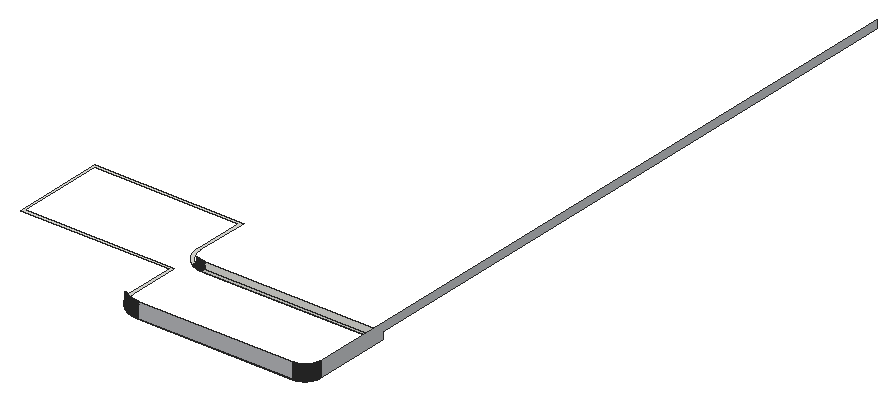
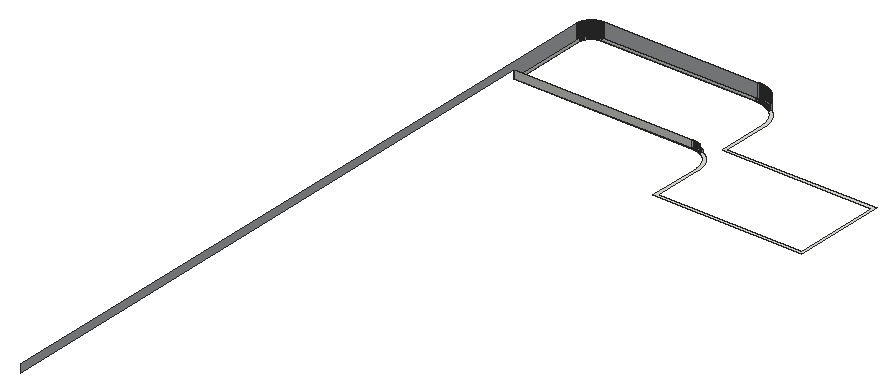
# SketchUp Ruby script. Lengths in inches.
U = 1.inch
M = Sketchup.active_model
def pt(a) = Geom::Point3d.new(a.map { |v| v * U })
def face(e, loops, mat)
  f = e.add_face(loops[0].map { |a| pt(a) })
  loops[1..].each { |l| e.add_face(l.map { |a| pt(a) }).erase! }
  f.material = f.back_material = mat if mat
  f
end
# faces: each face lists its corners as indices into pts; further lists are holes
def faces(e, pts, list, mat = nil) = list.each { |f| face(e, (f[0].is_a?(Array) ? f : [f]).map { |l| l.map { |i| pts[i] } }, mat) }
# xy, xz, yz: faces in a plane at the given z, y or x. An outline is a flat list of corners, or four numbers for a rectangle; further outlines are holes
def ring(l) = l.size == 4 ? [[l[0], l[1]], [l[2], l[1]], [l[2], l[3]], [l[0], l[3]]] : l.each_slice(2).to_a
def flat(e, list, mat, &to3) = list.each { |f| face(e, (f[0].is_a?(Array) ? f : [f]).map { |l| ring(l).map { |u, v| to3.(u, v) } }, mat) }
def xy(e, z, list, mat = nil) = flat(e, list, mat) { |x, y| [x, y, z] }
def xz(e, y, list, mat = nil) = flat(e, list, mat) { |x, z| [x, y, z] }
def yz(e, x, list, mat = nil) = flat(e, list, mat) { |y, z| [x, y, z] }
def lines(e, pts, list) = list.each { |a, b| e.add_line(pt(pts[a]), pt(pts[b])) }
# prism: a flat outline (further loops are holes) pulled along v
def prism(e, loops, v, mat = nil)
  f = face(e, loops, mat); d = Geom::Vector3d.new(v.map { |x| x * U })
  f.pushpull(f.normal.samedirection?(d) ? d.length : -d.length)
end
def box(e, o, s, mat = nil) = prism(e, [[o, [o[0] + s[0], o[1], o[2]], [o[0] + s[0], o[1] + s[1], o[2]], [o[0], o[1] + s[1], o[2]]]], [0, 0, s[2]], mat)
def at(x, y, z, deg = 0) = Geom::Transformation.translation(pt([x, y, z])) * Geom::Transformation.rotation(ORIGIN, Z_AXIS, deg.degrees)
def axes(o, x, y, z) = Geom::Transformation.new([*x, 0, *y, 0, *z, 0, *pt(o).to_a, 1])
def part(name) = M.definitions.add(name)
# library, detail: a bought-in or finely detailed component or shape, given as its bounding box
def library(name, o, s) = part(name).tap { |d| box(d.entities, o, s) }
def detail(e, o, s) = box(e.add_group.entities, o, s)
def put(e, d, t, mat = nil) = e.add_instance(d, t).tap { |i| i.material = mat if mat }
def group(e, t, mat = nil) = e.add_group.tap { |g| g.transformation = t; g.material = mat if mat }.entities
root = M.entities
M.materials.add("1427 AP 686 ARMOUR-N").color = [184, 186, 189]
xy(root,114,[[[157.6875,120,157.37,120.01,157.06,120.02,156.74,120.03,156.12,120.07,155.8,120.1,155.49,120.13,154.56,120.25,154.25,120.3,153.625,120.4,153.32,120.46,153.01,120.52,152.7,120.59,152.4,120.66,152.09,120.74,151.49,120.9,151.18,120.99,150.58,121.17,150.29,121.27,149.69,121.48,149.4,121.59,148.24,122.07,147.95,122.2,147.39,122.48,147.1,122.62,146.83,122.76,146.27,123.06,146,123.22,145.73,123.375,145.46,123.54,145.19,123.7,144.67,124.04,143.89,124.58,143.14,125.15,142.9,125.35,142.65,125.55,142.41,125.75,142.18,125.96,141.94,126.16,141.48,126.59,141.25,126.81,140.81,127.25,140.59,127.48,140.16,127.94,139.96,128.18,139.75,128.41,139.55,128.65,139.35,128.9,139.15,129.14,138.58,129.89,138.04,130.67,137.7,131.19,137.54,131.46,137.375,131.73,137.22,132,137.06,132.27,136.76,132.83,136.62,133.1,136.48,133.39,136.2,133.95,136.07,134.24,135.59,135.4,135.48,135.69,135.27,136.29,135.17,136.58,134.99,137.18,134.9,137.49,134.74,138.09,134.66,138.4,134.59,138.7,134.52,139.01,134.46,139.32,134.4,139.625,134.3,140.25,134.25,140.56,134.13,141.49,134.1,141.8,134.07,142.12,134.03,142.74,134.02,143.06,134.01,143.37,134,143.6875,134,180,18,180,18,252,134,252,134,209.78,134.01,209.57,134.01,209.35,134.03,208.91,134.05,208.7,134.0625,208.48,134.08,208.26,134.11,208.05,134.13,207.83,134.16,207.61,134.1875,207.4,134.22,207.18,134.26,206.97,134.29,206.76,134.34,206.54,134.42,206.12,134.47,205.9,134.52,205.69,134.58,205.48,134.63,205.27,134.69,205.0625,134.75,204.85,134.82,204.64,134.88,204.4375,134.95,204.23,135.02,204.03,135.09,203.82,135.17,203.62,135.25,203.41,135.41,203.01,135.5,202.8125,135.59,202.61,135.68,202.41,135.77,202.22,135.86,202.02,135.96,201.83,136.0625,201.63,136.16,201.44,136.27,201.25,136.48,200.875,136.6,200.6875,136.71,200.5,136.83,200.32,136.94,200.14,137.0625,199.95,137.1875,199.77,137.3125,199.6,137.4375,199.42,137.57,199.24,137.83,198.9,137.97,198.73,138.1,198.56,138.24,198.39,138.38,198.23,138.53,198.0625,138.67,197.9,138.97,197.58,139.12,197.43,139.27,197.27,139.43,197.12,139.58,196.97,139.9,196.67,140.0625,196.53,140.23,196.38,140.39,196.24,140.56,196.1,140.73,195.97,140.9,195.83,141.24,195.57,141.42,195.4375,141.6,195.3125,141.77,195.1875,141.95,195.0625,142.14,194.94,142.32,194.83,142.5,194.71,142.6875,194.6,142.875,194.48,143.25,194.27,143.44,194.16,143.63,194.0625,143.83,193.96,144.02,193.86,144.22,193.77,144.41,193.68,144.61,193.59,144.8125,193.5,145.01,193.41,145.41,193.25,145.62,193.17,145.82,193.09,146.03,193.02,146.23,192.95,146.4375,192.88,146.64,192.82,146.85,192.75,147.0625,192.69,147.27,192.63,147.48,192.58,147.69,192.52,147.9,192.47,148.12,192.42,148.54,192.34,148.76,192.29,148.97,192.26,149.18,192.22,149.4,192.1875,149.61,192.16,149.83,192.13,150.05,192.11,150.26,192.08,150.48,192.0625,150.7,192.05,150.91,192.03,151.35,192.01,151.57,192.01,151.78,192,290,192,290,131.76,289.99,131.53,289.98,131.29,289.96,131.06,289.94,130.82,289.92,130.59,289.89,130.36,289.85,130.12,289.8125,129.89,289.77,129.66,289.67,129.2,289.55,128.74,289.48,128.52,289.41,128.29,289.34,128.07,289.26,127.85,289.17,127.625,289.09,127.41,288.99,127.19,288.9,126.98,288.8,126.76,288.58,126.34,288.47,126.14,288.35,125.93,288.11,125.53,287.98,125.33,287.84,125.14,287.71,124.95,287.57,124.76,287.42,124.57,287.28,124.39,286.97,124.03,286.8125,123.85,286.65,123.68,286.49,123.51,286.32,123.35,286.15,123.1875,285.97,123.03,285.61,122.72,285.43,122.58,285.24,122.43,285.05,122.29,284.86,122.16,284.67,122.02,284.47,121.89,284.07,121.65,283.86,121.53,283.66,121.42,283.24,121.2,283.02,121.1,282.81,121.01,282.59,120.91,282.375,120.83,282.15,120.74,281.93,120.66,281.71,120.59,281.48,120.52,281.26,120.45,280.8,120.33,280.34,120.23,280.11,120.1875,279.88,120.15,279.64,120.11,279.41,120.08,279.18,120.06,278.94,120.04,278.71,120.02,278.47,120.01,278.24,120],[157.71,122,278.2,122,278.39,122.01,278.59,122.02,278.78,122.03,279.18,122.07,279.37,122.09,279.5625,122.125,279.76,122.16,279.95,122.19,280.14,122.23,280.33,122.28,280.52,122.32,280.9,122.43,281.28,122.55,281.46,122.62,281.64,122.6875,281.83,122.76,282.01,122.84,282.1875,122.92,282.36,123,282.54,123.09,282.71,123.18,282.89,123.28,283.06,123.37,283.22,123.47,283.56,123.69,283.88,123.91,284.04,124.03,284.34,124.27,284.49,124.4,284.64,124.52,284.79,124.66,284.93,124.79,285.21,125.07,285.34,125.21,285.73,125.66,285.97,125.96,286.09,126.12,286.31,126.44,286.53,126.78,286.63,126.94,286.72,127.11,286.82,127.29,286.91,127.46,287,127.64,287.08,127.8125,287.16,127.99,287.24,128.17,287.3125,128.36,287.38,128.54,287.45,128.72,287.57,129.1,287.68,129.48,287.72,129.67,287.77,129.86,287.81,130.05,287.84,130.24,287.875,130.4375,287.91,130.63,287.93,130.82,287.97,131.22,287.98,131.41,287.99,131.61,288,131.8,288,190,151.76,190,151.52,190.01,151.28,190.01,151.03,190.02,150.79,190.04,150.55,190.05,150.07,190.09,149.11,190.21,148.39,190.33,148.16,190.37,147.68,190.47,147.45,190.52,147.21,190.58,146.75,190.7,146.51,190.77,145.59,191.05,145.36,191.13,145.13,191.22,144.91,191.3,144.68,191.39,144.46,191.48,144.23,191.57,144.01,191.66,143.57,191.86,143.35,191.97,143.14,192.07,142.92,192.18,142.71,192.29,142.49,192.4,141.65,192.88,141.45,193.01,141.24,193.14,140.84,193.4,140.24,193.82,140.05,193.96,139.1,194.71,138.38,195.35,138.2,195.52,138.03,195.6875,137.86,195.86,137.6875,196.03,137.52,196.2,137.35,196.38,136.71,197.1,135.96,198.05,135.82,198.24,135.4,198.84,135.14,199.24,135.01,199.45,134.88,199.65,134.4,200.49,134.29,200.71,134.18,200.92,134.07,201.14,133.97,201.35,133.86,201.57,133.66,202.01,133.57,202.23,133.48,202.46,133.39,202.68,133.3,202.91,133.22,203.13,133.13,203.36,133.05,203.59,132.77,204.51,132.7,204.75,132.58,205.21,132.52,205.45,132.47,205.68,132.37,206.16,132.33,206.39,132.21,207.11,132.09,208.07,132.05,208.55,132.04,208.79,132.02,209.03,132.01,209.28,132.01,209.52,132,209.76,132,250,20,250,20,182,136,182,136,143.71,136.01,143.42,136.02,143.14,136.03,142.85,136.05,142.5625,136.07,142.27,136.09,141.99,136.15,141.41,136.1875,141.13,136.23,140.84,136.27,140.56,136.32,140.27,136.42,139.71,136.48,139.43,136.54,139.14,136.68,138.58,136.75,138.31,136.91,137.75,136.99,137.48,137.08,137.2,137.26,136.66,137.46,136.12,137.57,135.85,137.67,135.58,137.79,135.32,137.9,135.05,138.14,134.53,138.4,134.01,138.53,133.76,138.67,133.5,139.09,132.75,139.24,132.51,139.39,132.26,140.03,131.3,140.37,130.84,140.55,130.61,140.72,130.38,140.9,130.15,141.09,129.93,141.27,129.71,141.46,129.49,141.84,129.07,142.44,128.44,143.07,127.84,143.49,127.46,143.71,127.27,143.93,127.09,144.15,126.9,144.38,126.72,144.61,126.55,144.84,126.37,145.3,126.03,146.26,125.39,146.51,125.24,146.75,125.09,147.5,124.67,147.76,124.53,148.01,124.4,148.53,124.14,149.05,123.9,149.32,123.79,149.58,123.67,149.85,123.57,150.12,123.46,150.66,123.26,151.2,123.08,151.48,122.99,151.75,122.91,152.31,122.75,152.58,122.68,153.14,122.54,153.43,122.48,153.71,122.42,154.27,122.32,154.56,122.27,154.84,122.23,155.13,122.1875,155.41,122.15,155.99,122.09,156.27,122.07,156.5625,122.05,156.85,122.03,157.14,122.02,157.42,122.01]]])
xz(root,120,[[157.6875,114,158,126],[158,114,278,126],[278,114,278.24,126]],"1427 AP 686 ARMOUR-N")
xz(root,122,[[157.71,114,158,116],[158,114,278,116],[278,114,278.2,116]])
xz(root,190,[[151.76,114,151.97,116],[151.97,114,152,116],[152,114,288,116]])
xz(root,190.01,[[151.28,114,151.52,116]])
xz(root,192,[[151.78,114,151.97,120],[151.97,114,152,120],[152,114,290,120]])
xz(root,192.01,[[151.35,114,151.57,120]])
yz(root,288,[[131.8,114,132,116],[132,114,190,116]])
yz(root,290,[[131.76,114,132,126],[132,114,192,114,192,120,672,120,672,126,132,126]],"1427 AP 686 ARMOUR-N")
p = [[156.74,120.03,126],[156.43,120.05,126],[156.43,120.05,114],[156.74,120.03,114],[157.06,120.02,126],[157.06,120.02,114],
  [157.37,120.01,126],[157.37,120.01,114],[157.6875,120,126],[157.6875,120,114],[278.47,120.01,126],[278.24,120,126],
  [278.24,120,114],[278.47,120.01,114],[278.71,120.02,126],[278.71,120.02,114],[278.94,120.04,126],[278.94,120.04,114],
  [279.18,120.06,126],[279.18,120.06,114],[155.49,120.13,126],[155.18,120.17,126],[155.18,120.17,114],[155.49,120.13,114],
  [155.8,120.1,126],[155.8,120.1,114],[156.12,120.07,126],[156.12,120.07,114],[279.41,120.08,126],[279.41,120.08,114],
  [279.64,120.11,126],[279.64,120.11,114],[279.88,120.15,126],[279.88,120.15,114],[280.11,120.1875,126],[280.11,120.1875,114],
  [154.56,120.25,126],[154.25,120.3,126],[154.25,120.3,114],[154.56,120.25,114],[154.87,120.21,126],[154.87,120.21,114],
  [280.34,120.23,126],[280.34,120.23,114],[280.57,120.28,126],[280.57,120.28,114],[153.9375,120.35,126],[153.625,120.4,126],
  [153.625,120.4,114],[153.9375,120.35,114],[280.8,120.33,126],[280.8,120.33,114],[281.03,120.39,126],[281.03,120.39,114],
  [153.32,120.46,126],[153.32,120.46,114],[281.26,120.45,126],[281.26,120.45,114],[153.01,120.52,126],[152.7,120.59,126],
  [152.7,120.59,114],[153.01,120.52,114],[281.48,120.52,126],[281.48,120.52,114],[281.71,120.59,126],[281.71,120.59,114],
  [152.4,120.66,126],[152.4,120.66,114],[281.93,120.66,126],[281.93,120.66,114],[152.09,120.74,126],[151.79,120.82,126],
  [151.79,120.82,114],[152.09,120.74,114],[282.15,120.74,126],[282.15,120.74,114],[282.375,120.83,126],[282.375,120.83,114],
  [151.49,120.9,126],[151.49,120.9,114],[282.59,120.91,126],[282.59,120.91,114],[151.18,120.99,126],[151.18,120.99,114],
  [282.81,121.01,126],[282.81,121.01,114],[150.88,121.08,126],[150.88,121.08,114],[283.02,121.1,126],[283.02,121.1,114],
  [150.58,121.17,126],[150.58,121.17,114],[283.24,121.2,126],[283.24,121.2,114],[150.29,121.27,126],[150.29,121.27,114],
  [283.45,121.31,126],[283.45,121.31,114],[149.99,121.375,126],[149.99,121.375,114],[283.66,121.42,126],[283.66,121.42,114],
  [149.69,121.48,126],[149.69,121.48,114],[283.86,121.53,126],[283.86,121.53,114],[149.4,121.59,126],[149.4,121.59,114],
  [284.07,121.65,126],[284.07,121.65,114],[149.11,121.71,126],[149.11,121.71,114],[284.27,121.77,126],[284.27,121.77,114],
  [148.82,121.83,126],[148.82,121.83,114],[148.53,121.95,126],[148.53,121.95,114],[284.47,121.89,126],[284.47,121.89,114],
  [148.24,122.07,126],[148.24,122.07,114],[284.67,122.02,126],[284.67,122.02,114],[156.5625,122.05,114],[156.27,122.07,114],
  [156.27,122.07,116],[156.5625,122.05,116],[156.85,122.03,114],[156.85,122.03,116],[157.14,122.02,114],[157.14,122.02,116],
  [157.42,122.01,114],[157.42,122.01,116],[157.71,122,114],[157.71,122,116],[278.39,122.01,114],[278.2,122,114],
  [278.2,122,116],[278.39,122.01,116],[278.59,122.02,114],[278.59,122.02,116],[278.78,122.03,114],[278.78,122.03,116],
  [278.98,122.05,114],[278.98,122.05,116],[279.18,122.07,114],[279.18,122.07,116],[284.86,122.16,126],[284.86,122.16,114],
  [147.95,122.2,126],[147.95,122.2,114],[155.7,122.12,114],[155.41,122.15,114],[155.41,122.15,116],[155.7,122.12,116],
  [155.99,122.09,114],[155.99,122.09,116],[279.37,122.09,114],[279.37,122.09,116],[279.5625,122.125,114],[279.5625,122.125,116],
  [279.76,122.16,114],[279.76,122.16,116],[147.67,122.34,126],[147.67,122.34,114],[154.84,122.23,114],[154.56,122.27,114],
  [154.56,122.27,116],[154.84,122.23,116],[155.13,122.1875,114],[155.13,122.1875,116],[279.95,122.19,114],[279.95,122.19,116],
  [280.14,122.23,114],[280.14,122.23,116],[280.33,122.28,114],[280.33,122.28,116],[285.05,122.29,126],[285.05,122.29,114],
  [147.39,122.48,126],[147.39,122.48,114],[154.27,122.32,114],[153.99,122.37,114],[153.99,122.37,116],[154.27,122.32,116],
  [280.52,122.32,114],[280.52,122.32,116],[280.71,122.375,114],[280.71,122.375,116],[285.24,122.43,126],[285.24,122.43,114],
  [153.71,122.42,114],[153.43,122.48,114],[153.43,122.48,116],[153.71,122.42,116],[280.9,122.43,114],[280.9,122.43,116],
  [281.09,122.49,114],[281.09,122.49,116],[285.43,122.58,126],[285.43,122.58,114],[147.1,122.62,126],[147.1,122.62,114],
  [153.14,122.54,114],[152.86,122.61,114],[152.86,122.61,116],[153.14,122.54,116],[281.28,122.55,114],[281.28,122.55,116],
  [146.83,122.76,126],[146.83,122.76,114],[152.58,122.68,114],[152.58,122.68,116],[281.46,122.62,114],[281.46,122.62,116],
  [281.64,122.6875,114],[281.64,122.6875,116],[285.61,122.72,126],[285.61,122.72,114],[152.31,122.75,114],[152.03,122.83,114],
  [152.03,122.83,116],[152.31,122.75,116],[281.83,122.76,114],[281.83,122.76,116],[285.79,122.875,126],[285.79,122.875,114],
  [146.55,122.91,126],[146.55,122.91,114],[151.75,122.91,114],[151.75,122.91,116],[282.01,122.84,114],[282.01,122.84,116],
  [282.1875,122.92,114],[282.1875,122.92,116],[146.27,123.06,126],[146.27,123.06,114],[151.48,122.99,114],[151.48,122.99,116],
  [282.36,123,114],[282.36,123,116],[285.97,123.03,126],[285.97,123.03,114],[151.2,123.08,114],[151.2,123.08,116],
  [282.54,123.09,114],[282.54,123.09,116],[286.15,123.1875,126],[286.15,123.1875,114],[146,123.22,126],[146,123.22,114],
  [150.93,123.17,114],[150.93,123.17,116],[282.71,123.18,114],[282.71,123.18,116],[145.73,123.375,126],[145.73,123.375,114],
  [150.66,123.26,114],[150.66,123.26,116],[282.89,123.28,114],[282.89,123.28,116],[286.32,123.35,126],[286.32,123.35,114],
  [150.39,123.36,114],[150.39,123.36,116],[283.06,123.37,114],[283.06,123.37,116],[286.49,123.51,126],[286.49,123.51,114],
  [145.46,123.54,126],[145.46,123.54,114],[150.12,123.46,114],[150.12,123.46,116],[283.22,123.47,114],[283.22,123.47,116],
  [145.19,123.7,126],[145.19,123.7,114],[149.85,123.57,114],[149.85,123.57,116],[283.39,123.58,114],[283.39,123.58,116],
  [286.65,123.68,126],[286.65,123.68,114],[149.58,123.67,114],[149.58,123.67,116],[283.56,123.69,114],[283.56,123.69,116],
  [144.93,123.87,126],[144.93,123.87,114],[149.32,123.79,114],[149.32,123.79,116],[283.72,123.8,114],[283.72,123.8,116],
  [286.8125,123.85,126],[286.8125,123.85,114],[149.05,123.9,114],[149.05,123.9,116],[283.88,123.91,114],[283.88,123.91,116],
  [144.67,124.04,126],[144.67,124.04,114],[148.79,124.02,114],[148.79,124.02,116],[284.04,124.03,114],[284.04,124.03,116],
  [286.97,124.03,126],[286.97,124.03,114],[144.41,124.22,126],[144.41,124.22,114],[148.53,124.14,114],[148.53,124.14,116],
  [284.19,124.15,114],[284.19,124.15,116],[287.125,124.21,126],[287.125,124.21,114],[148.27,124.27,114],[148.27,124.27,116],
  [284.34,124.27,114],[284.34,124.27,116],[144.15,124.4,126],[144.15,124.4,114],[287.28,124.39,126],[287.28,124.39,114],
  [148.01,124.4,114],[148.01,124.4,116],[284.49,124.4,114],[284.49,124.4,116],[143.89,124.58,126],[143.89,124.58,114],
  [147.76,124.53,114],[147.76,124.53,116],[284.64,124.52,114],[284.64,124.52,116],[287.42,124.57,126],[287.42,124.57,114],
  [147.5,124.67,114],[147.5,124.67,116],[284.79,124.66,114],[284.79,124.66,116],[287.57,124.76,126],[287.57,124.76,114],
  [147.25,124.81,114],[147.25,124.81,116],[284.93,124.79,114],[284.93,124.79,116],[147,124.95,114],[147,124.95,116],
  [285.07,124.93,114],[285.07,124.93,116],[287.71,124.95,126],[287.71,124.95,114],[146.75,125.09,114],[146.75,125.09,116],
  [285.21,125.07,114],[285.21,125.07,116],[287.84,125.14,126],[287.84,125.14,114],[146.51,125.24,114],[146.51,125.24,116],
  [285.34,125.21,114],[285.34,125.21,116],[287.98,125.33,126],[287.98,125.33,114],[146.26,125.39,114],[146.26,125.39,116],
  [285.47,125.36,114],[285.47,125.36,116],[288.11,125.53,126],[288.11,125.53,114],[146.02,125.55,114],[146.02,125.55,116],
  [285.6,125.51,114],[285.6,125.51,116],[145.78,125.71,114],[145.78,125.71,116],[285.73,125.66,114],[285.73,125.66,116],
  [288.23,125.73,126],[288.23,125.73,114],[145.54,125.87,114],[145.54,125.87,116],[285.85,125.81,114],[285.85,125.81,116],
  [288.35,125.93,126],[288.35,125.93,114],[285.97,125.96,114],[285.97,125.96,116],[145.3,126.03,114],[145.3,126.03,116],
  [288.47,126.14,126],[288.47,126.14,114],[145.07,126.2,114],[145.07,126.2,116],[286.09,126.12,114],[286.09,126.12,116],
  [286.2,126.28,114],[286.2,126.28,116],[288.58,126.34,126],[288.58,126.34,114],[144.84,126.37,114],[144.84,126.37,116],
  [286.31,126.44,114],[286.31,126.44,116],[288.69,126.55,126],[288.69,126.55,114],[144.61,126.55,114],[144.61,126.55,116],
  [286.42,126.61,114],[286.42,126.61,116],[144.38,126.72,114],[144.38,126.72,116],[286.53,126.78,114],[286.53,126.78,116],
  [288.8,126.76,126],[288.8,126.76,114],[144.15,126.9,114],[144.15,126.9,116],[286.63,126.94,114],[286.63,126.94,116],
  [288.9,126.98,126],[288.9,126.98,114],[143.93,127.09,114],[143.93,127.09,116],[286.72,127.11,114],[286.72,127.11,116],
  [288.99,127.19,126],[288.99,127.19,114],[143.71,127.27,114],[143.71,127.27,116],[286.82,127.29,114],[286.82,127.29,116],
  [289.09,127.41,126],[289.09,127.41,114],[286.91,127.46,114],[286.91,127.46,116],[289.17,127.625,126],[289.17,127.625,114],
  [287,127.64,114],[287,127.64,116],[287.08,127.8125,114],[287.08,127.8125,116],[289.26,127.85,126],[289.26,127.85,114],
  [287.16,127.99,114],[287.16,127.99,116],[289.34,128.07,126],[289.34,128.07,114],[287.24,128.17,114],[287.24,128.17,116],
  [289.41,128.29,126],[289.41,128.29,114],[287.3125,128.36,114],[287.3125,128.36,116],[289.48,128.52,126],[289.48,128.52,114],
  [287.38,128.54,114],[287.38,128.54,116],[287.45,128.72,114],[287.45,128.72,116],[289.55,128.74,126],[289.55,128.74,114],
  [287.51,128.91,114],[287.51,128.91,116],[289.61,128.97,126],[289.61,128.97,114],[287.57,129.1,114],[287.57,129.1,116],
  [289.67,129.2,126],[289.67,129.2,114],[287.625,129.29,114],[287.625,129.29,116],[289.72,129.43,126],[289.72,129.43,114],
  [287.68,129.48,114],[287.68,129.48,116],[289.77,129.66,126],[289.77,129.66,114],[287.72,129.67,114],[287.72,129.67,116],
  [287.77,129.86,114],[287.77,129.86,116],[289.8125,129.89,126],[289.8125,129.89,114],[287.81,130.05,114],[287.81,130.05,116],
  [289.85,130.12,126],[289.85,130.12,114],[287.84,130.24,114],[287.84,130.24,116],[289.89,130.36,126],[289.89,130.36,114],
  [287.875,130.4375,114],[287.875,130.4375,116],[287.91,130.63,114],[287.91,130.63,116],[289.92,130.59,126],[289.92,130.59,114],
  [287.93,130.82,114],[287.93,130.82,116],[289.94,130.82,126],[289.94,130.82,114],[287.95,131.02,114],[287.95,131.02,116],
  [289.96,131.06,126],[289.96,131.06,114],[287.97,131.22,114],[287.97,131.22,116],[289.98,131.29,126],[289.98,131.29,114],
  [287.98,131.41,114],[287.98,131.41,116],[289.99,131.53,126],[289.99,131.53,114],[287.99,131.61,114],[287.99,131.61,116],
  [290,131.76,126],[290,131.76,114],[288,131.8,114],[288,131.8,116],[150.55,190.05,114],[150.79,190.04,114],
  [150.79,190.04,116],[150.55,190.05,116],[151.03,190.02,114],[151.03,190.02,116],[151.28,190.01,114],[151.28,190.01,116],
  [151.52,190.01,114],[151.76,190,114],[151.76,190,116],[151.52,190.01,116],[149.35,190.18,114],[149.59,190.15,114],
  [149.59,190.15,116],[149.35,190.18,116],[149.83,190.12,114],[149.83,190.12,116],[150.07,190.09,114],[150.07,190.09,116],
  [150.31,190.07,114],[150.31,190.07,116],[148.63,190.29,114],[148.87,190.25,114],[148.87,190.25,116],[148.63,190.29,116],
  [149.11,190.21,114],[149.11,190.21,116],[148.16,190.37,114],[148.39,190.33,114],[148.39,190.33,116],[148.16,190.37,116],
  [147.68,190.47,114],[147.92,190.42,114],[147.92,190.42,116],[147.68,190.47,116],[147.21,190.58,114],[147.45,190.52,114],
  [147.45,190.52,116],[147.21,190.58,116],[146.75,190.7,114],[146.98,190.64,114],[146.98,190.64,116],[146.75,190.7,116],
  [146.51,190.77,114],[146.51,190.77,116],[146.05,190.91,114],[146.28,190.84,114],[146.28,190.84,116],[146.05,190.91,116],
  [145.82,190.98,114],[145.82,190.98,116],[145.59,191.05,114],[145.59,191.05,116],[145.13,191.22,114],[145.36,191.13,114],
  [145.36,191.13,116],[145.13,191.22,116],[144.91,191.3,114],[144.91,191.3,116],[144.68,191.39,114],[144.68,191.39,116],
  [144.46,191.48,114],[144.46,191.48,116],[144.23,191.57,114],[144.23,191.57,116],[144.01,191.66,114],[144.01,191.66,116],
  [143.79,191.76,114],[143.79,191.76,116],[150.48,192.0625,120],[150.7,192.05,120],[150.7,192.05,114],[150.48,192.0625,114],
  [150.91,192.03,120],[150.91,192.03,114],[151.13,192.02,120],[151.13,192.02,114],[151.35,192.01,120],[151.35,192.01,114],
  [151.57,192.01,120],[151.78,192,120],[151.78,192,114],[151.57,192.01,114],[149.61,192.16,120],[149.83,192.13,120],
  [149.83,192.13,114],[149.61,192.16,114],[150.05,192.11,120],[150.05,192.11,114],[150.26,192.08,120],[150.26,192.08,114],
  [148.97,192.26,120],[149.18,192.22,120],[149.18,192.22,114],[148.97,192.26,114],[149.4,192.1875,120],[149.4,192.1875,114],
  [148.33,192.38,120],[148.54,192.34,120],[148.54,192.34,114],[148.33,192.38,114],[148.76,192.29,120],[148.76,192.29,114],
  [147.9,192.47,120],[148.12,192.42,120],[148.12,192.42,114],[147.9,192.47,114],[147.48,192.58,120],[147.69,192.52,120],
  [147.69,192.52,114],[147.48,192.58,114],[147.0625,192.69,120],[147.27,192.63,120],[147.27,192.63,114],[147.0625,192.69,114],
  [146.85,192.75,120],[146.85,192.75,114],[146.4375,192.88,120],[146.64,192.82,120],[146.64,192.82,114],[146.4375,192.88,114],
  [146.03,193.02,120],[146.23,192.95,120],[146.23,192.95,114],[146.03,193.02,114],[145.82,193.09,120],[145.82,193.09,114],
  [145.62,193.17,120],[145.62,193.17,114],[145.21,193.33,120],[145.41,193.25,120],[145.41,193.25,114],[145.21,193.33,114],
  [145.01,193.41,120],[145.01,193.41,114],[144.8125,193.5,120],[144.8125,193.5,114],[144.61,193.59,120],[144.61,193.59,114],
  [144.41,193.68,120],[144.41,193.68,114],[144.22,193.77,120],[144.22,193.77,114],[144.02,193.86,120],[144.02,193.86,114],
  [143.83,193.96,120],[143.83,193.96,114]]
faces(root,p,[[0,1,2,3],[4,0,3,5],[6,4,5,7],[8,6,7,9],[10,11,12,13],[14,10,13,15],[16,14,15,17],[18,16,17,19],
  [20,21,22,23],[24,20,23,25],[26,24,25,27],[1,26,27,2],[28,18,19,29],[30,28,29,31],[32,30,31,33],[34,32,33,35],
  [36,37,38,39],[40,36,39,41],[21,40,41,22],[42,34,35,43],[44,42,43,45],[46,47,48,49],[37,46,49,38],[50,44,45,51],
  [52,50,51,53],[47,54,55,48],[56,52,53,57],[58,59,60,61],[54,58,61,55],[62,56,57,63],[64,62,63,65],[59,66,67,60],
  [68,64,65,69],[70,71,72,73],[66,70,73,67],[74,68,69,75],[76,74,75,77],[71,78,79,72],[80,76,77,81],[78,82,83,79],
  [84,80,81,85],[82,86,87,83],[88,84,85,89],[86,90,91,87],[92,88,89,93],[90,94,95,91],[96,92,93,97],[94,98,99,95],
  [100,96,97,101],[98,102,103,99],[104,100,101,105],[102,106,107,103],[108,104,105,109],[106,110,111,107],[112,108,109,113],[110,114,115,111],
  [114,116,117,115],[118,112,113,119],[116,120,121,117],[122,118,119,123],[148,122,123,149],[120,150,151,121],[150,164,165,151],[178,148,149,179],
  [164,180,181,165],[190,178,179,191],[200,190,191,201],[180,202,203,181],[202,210,211,203],[218,200,201,219],[226,218,219,227],[210,228,229,211],
  [228,236,237,229],[242,226,227,243],[248,242,243,249],[236,250,251,237],[250,256,257,251],[262,248,249,263],[268,262,263,269],[256,270,271,257],
  [270,276,277,271],[282,268,269,283],[276,288,289,277],[294,282,283,295],[288,300,301,289],[306,294,295,307],[300,308,309,301],[314,306,307,315],
  [308,320,321,309],[322,314,315,323],[320,328,329,321],[334,322,323,335],[340,334,335,341],[350,340,341,351],[356,350,351,357],[362,356,357,363],
  [368,362,363,369],[378,368,369,379],[384,378,379,385],[390,384,385,391],[398,390,391,399],[404,398,399,405],[414,404,405,415],[420,414,415,421],
  [426,420,421,427],[432,426,427,433],[436,432,433,437],[442,436,437,443],[446,442,443,447],[450,446,447,451],[454,450,451,455],[460,454,455,461],
  [464,460,461,465],[468,464,465,469],[472,468,469,473],[476,472,473,477],[482,476,477,483],[486,482,483,487],[490,486,487,491],[496,490,491,497],
  [500,496,497,501],[504,500,501,505],[508,504,505,509],[512,508,509,513],[516,512,513,517]],"1427 AP 686 ARMOUR-N")
faces(root,p,[[124,125,126,127],[128,124,127,129],[130,128,129,131],[132,130,131,133],[134,132,133,135],[136,137,138,139],[140,136,139,141],[142,140,141,143],
  [144,142,143,145],[146,144,145,147],[152,153,154,155],[156,152,155,157],[125,156,157,126],[158,146,147,159],[160,158,159,161],[162,160,161,163],
  [166,167,168,169],[170,166,169,171],[153,170,171,154],[172,162,163,173],[174,172,173,175],[176,174,175,177],[182,183,184,185],[167,182,185,168],
  [186,176,177,187],[188,186,187,189],[192,193,194,195],[183,192,195,184],[196,188,189,197],[198,196,197,199],[204,205,206,207],[193,204,207,194],
  [208,198,199,209],[205,212,213,206],[214,208,209,215],[216,214,215,217],[220,221,222,223],[212,220,223,213],[224,216,217,225],[221,230,231,222],
  [232,224,225,233],[234,232,233,235],[230,238,239,231],[240,234,235,241],[238,244,245,239],[246,240,241,247],[244,252,253,245],[254,246,247,255],
  [252,258,259,253],[260,254,255,261],[258,264,265,259],[266,260,261,267],[264,272,273,265],[274,266,267,275],[272,278,279,273],[280,274,275,281],
  [278,284,285,279],[286,280,281,287],[284,290,291,285],[292,286,287,293],[290,296,297,291],[298,292,293,299],[296,302,303,297],[304,298,299,305],
  [302,310,311,303],[312,304,305,313],[310,316,317,311],[318,312,313,319],[316,324,325,317],[326,318,319,327],[324,330,331,325],[332,326,327,333],
  [330,336,337,331],[338,332,333,339],[336,342,343,337],[344,338,339,345],[342,346,347,343],[348,344,345,349],[346,352,353,347],[354,348,349,355],
  [352,358,359,353],[360,354,355,361],[358,364,365,359],[366,360,361,367],[364,370,371,365],[372,366,367,373],[370,374,375,371],[376,372,373,377],
  [374,380,381,375],[382,376,377,383],[386,382,383,387],[380,388,389,381],[388,392,393,389],[394,386,387,395],[396,394,395,397],[392,400,401,393],
  [402,396,397,403],[400,406,407,401],[408,402,403,409],[406,410,411,407],[412,408,409,413],[410,416,417,411],[418,412,413,419],[416,422,423,417],
  [424,418,419,425],[422,428,429,423],[430,424,425,431],[434,430,431,435],[438,434,435,439],[440,438,439,441],[444,440,441,445],[448,444,445,449],
  [452,448,449,453],[456,452,453,457],[458,456,457,459],[462,458,459,463],[466,462,463,467],[470,466,467,471],[474,470,471,475],[478,474,475,479],
  [480,478,479,481],[484,480,481,485],[488,484,485,489],[492,488,489,493],[494,492,493,495],[498,494,495,499],[502,498,499,503],[506,502,503,507],
  [510,506,507,511],[514,510,511,515],[518,514,515,519],[520,521,522,523],[521,524,525,522],[524,526,527,525],[528,529,530,531],[532,533,534,535],
  [533,536,537,534],[536,538,539,537],[538,540,541,539],[540,520,523,541],[542,543,544,545],[543,546,547,544],[546,532,535,547],[548,549,550,551],
  [549,542,545,550],[552,553,554,555],[553,548,551,554],[556,557,558,559],[557,552,555,558],[560,561,562,563],[561,556,559,562],[564,560,563,565],
  [566,567,568,569],[567,564,565,568],[570,566,569,571],[572,570,571,573],[574,575,576,577],[575,572,573,576],[578,574,577,579],[580,578,579,581],
  [582,580,581,583],[584,582,583,585],[586,584,585,587],[588,586,587,589],[590,591,592,593],[591,594,595,592],[594,596,597,595],[596,598,599,597],
  [600,601,602,603],[604,605,606,607],[605,608,609,606],[608,610,611,609],[610,590,593,611],[612,613,614,615],[613,616,617,614],[616,604,607,617],
  [618,619,620,621],[619,622,623,620],[622,612,615,623],[624,625,626,627],[625,618,621,626],[628,629,630,631],[629,624,627,630],[632,633,634,635],
  [633,628,631,634],[636,632,635,637],[638,639,640,641],[639,636,637,640],[642,643,644,645],[643,638,641,644],[646,642,645,647],[648,646,647,649],
  [650,651,652,653],[651,648,649,652],[654,650,653,655],[656,654,655,657],[658,656,657,659],[660,658,659,661],[662,660,661,663],[664,662,663,665],
  [666,664,665,667]])
